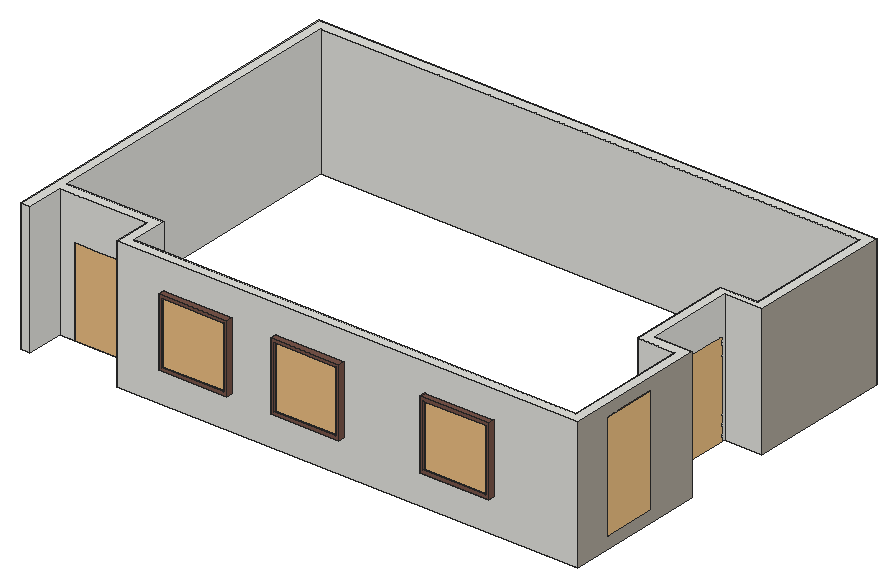
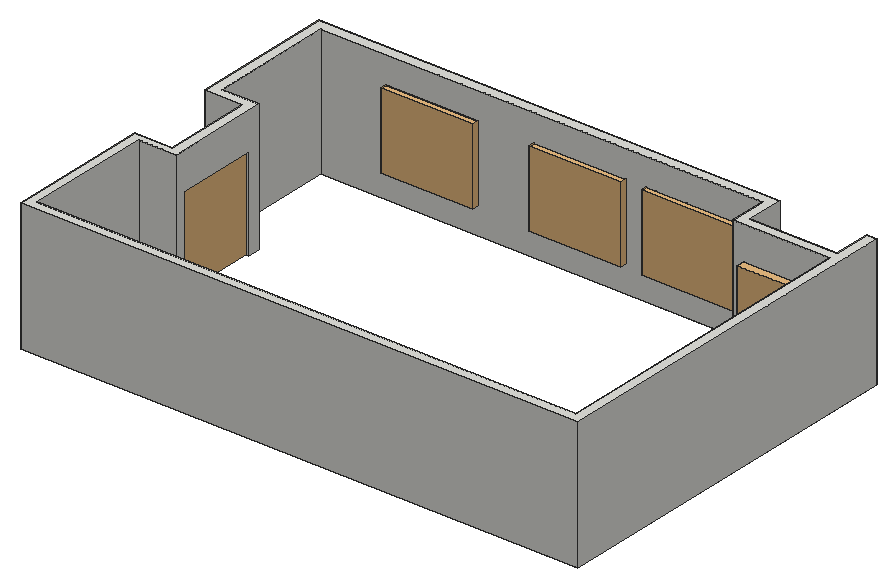
# SketchUp Ruby script. Lengths in inches.
U = 1.inch
M = Sketchup.active_model
def pt(a) = Geom::Point3d.new(a.map { |v| v * U })
def face(e, loops, mat)
  f = e.add_face(loops[0].map { |a| pt(a) })
  loops[1..].each { |l| e.add_face(l.map { |a| pt(a) }).erase! }
  f.material = f.back_material = mat if mat
  f
end
# faces: each face lists its corners as indices into pts; further lists are holes
def faces(e, pts, list, mat = nil) = list.each { |f| face(e, (f[0].is_a?(Array) ? f : [f]).map { |l| l.map { |i| pts[i] } }, mat) }
# xy, xz, yz: faces in a plane at the given z, y or x. An outline is a flat list of corners, or four numbers for a rectangle; further outlines are holes
def ring(l) = l.size == 4 ? [[l[0], l[1]], [l[2], l[1]], [l[2], l[3]], [l[0], l[3]]] : l.each_slice(2).to_a
def flat(e, list, mat, &to3) = list.each { |f| face(e, (f[0].is_a?(Array) ? f : [f]).map { |l| ring(l).map { |u, v| to3.(u, v) } }, mat) }
def xy(e, z, list, mat = nil) = flat(e, list, mat) { |x, y| [x, y, z] }
def xz(e, y, list, mat = nil) = flat(e, list, mat) { |x, z| [x, y, z] }
def yz(e, x, list, mat = nil) = flat(e, list, mat) { |y, z| [x, y, z] }
def lines(e, pts, list) = list.each { |a, b| e.add_line(pt(pts[a]), pt(pts[b])) }
# prism: a flat outline (further loops are holes) pulled along v
def prism(e, loops, v, mat = nil)
  f = face(e, loops, mat); d = Geom::Vector3d.new(v.map { |x| x * U })
  f.pushpull(f.normal.samedirection?(d) ? d.length : -d.length)
end
def box(e, o, s, mat = nil) = prism(e, [[o, [o[0] + s[0], o[1], o[2]], [o[0] + s[0], o[1] + s[1], o[2]], [o[0], o[1] + s[1], o[2]]]], [0, 0, s[2]], mat)
def at(x, y, z, deg = 0) = Geom::Transformation.translation(pt([x, y, z])) * Geom::Transformation.rotation(ORIGIN, Z_AXIS, deg.degrees)
def axes(o, x, y, z) = Geom::Transformation.new([*x, 0, *y, 0, *z, 0, *pt(o).to_a, 1])
def part(name) = M.definitions.add(name)
# library, detail: a bought-in or finely detailed component or shape, given as its bounding box
def library(name, o, s) = part(name).tap { |d| box(d.entities, o, s) }
def detail(e, o, s) = box(e.add_group.entities, o, s)
def put(e, d, t, mat = nil) = e.add_instance(d, t).tap { |i| i.material = mat if mat }
def group(e, t, mat = nil) = e.add_group.tap { |g| g.transformation = t; g.material = mat if mat }.entities
root = M.entities
M.materials.add("1111 AP 9939 Brown seed-N").color = [120, 84, 73]
M.materials.add("Generic").color = [172, 166, 153]
M.materials.add("[Granite Dark Gray]").color = [69, 68, 68]
M.materials.add("[Wood Veneer 01]").color = [120, 70, 37]
c1 = library("Double-hung window 69 in. x 58 in. triple row with mullions",[0,0,-3.59],[62,58,4.59])
c2 = library("Glass Door",[0,0,0],[72,3.54,96])
c3 = library("RIDEAUX \#16",[0,0,0],[103.86,7.74,93.57])
c4 = library("Curtain",[0,0,0],[121.12,7.86,100.24])
c5 = library("SLIDING+GLASS+DOOR",[0,-0.75,0],[72,5.75,80])
c6 = library("Group\#21",[0,0,0],[0.5,51,102])
g1 = group(root,at(36,101.37,167.79))
xy(g1,0,[[0,6,0,366,537,366,537,228,501,228,501,225,492,225,492,234,528,234,528,357,9,357,9,51,24,51,24,42,9,42,9,6],[93,6,93,42,78,42,78,51,102,51,102,15,528,15,528,135,492,135,492,147,501,147,501,144,537,144,537,6]])
xy(g1,33,[[138,0,204,6],[246,0,312,6],[390,0,456,6]],"1111 AP 9939 Brown seed-N")
xy(g1,36,[[141,0,201,15],[249,0,309,15],[393,0,453,15]],"1111 AP 9939 Brown seed-N")
xy(g1,84,[[24,42,78,51]])
xy(g1,90,[[492,147,501,225]])
xy(g1,96,[[141,0,201,15],[249,0,309,15],[393,0,453,15]],"1111 AP 9939 Brown seed-N")
xy(g1,99,[[138,0,204,6],[246,0,312,6],[390,0,456,6]],"1111 AP 9939 Brown seed-N")
xy(g1,126,[[[0,6,9,6,9,42,93,42,93,6,537,6,537,144,501,144,501,228,537,228,537,366,0,366],[102,15,102,51,9,51,9,357,528,357,528,234,492,234,492,135,528,135,528,15]]])
xz(g1,0,[[[138,33,204,99],[141,36,201,96]],[[246,33,312,99],[249,36,309,96]],[[390,33,456,99],[393,36,453,96]]],"1111 AP 9939 Brown seed-N")
xz(g1,6,[[0,0,9,126],[[93,0,537,126],[138,33,204,99],[246,33,312,99],[390,33,456,99]]])
xz(g1,15,[[[102,0,528,126],[141,36,201,96],[249,36,309,96],[393,36,453,96]]])
xz(g1,42,[[9,0,24,0,24,84,78,84,78,0,93,0,93,126,9,126]])
xz(g1,51,[[9,0,9,126,102,126,102,0,78,0,78,84,24,84,24,0]])
xz(g1,135,[[492,0,528,126]])
xz(g1,144,[[501,0,537,126]])
xz(g1,147,[[492,0,501,90]])
xz(g1,225,[[492,0,501,90]])
xz(g1,228,[[501,0,537,126]])
xz(g1,234,[[492,0,528,126]])
xz(g1,357,[[9,0,528,126]])
xz(g1,366,[[0,0,537,126]])
yz(g1,0,[[6,0,366,126]])
yz(g1,9,[[6,0,42,126],[51,0,357,126]])
yz(g1,24,[[42,0,51,84]])
yz(g1,78,[[42,0,51,84]])
yz(g1,93,[[6,0,42,126]])
yz(g1,102,[[15,0,51,126]])
yz(g1,138,[[0,33,6,99]],"[Wood Veneer 01]")
yz(g1,141,[[0,36,15,96]],"1111 AP 9939 Brown seed-N")
yz(g1,201,[[0,36,15,96]],"1111 AP 9939 Brown seed-N")
yz(g1,204,[[0,33,6,99]],"1111 AP 9939 Brown seed-N")
yz(g1,246,[[0,33,6,99]],"1111 AP 9939 Brown seed-N")
yz(g1,249,[[0,36,15,96]],"1111 AP 9939 Brown seed-N")
yz(g1,309,[[0,36,15,96]],"1111 AP 9939 Brown seed-N")
yz(g1,312,[[0,33,6,99]],"1111 AP 9939 Brown seed-N")
yz(g1,390,[[0,33,6,99]],"1111 AP 9939 Brown seed-N")
yz(g1,393,[[0,36,15,96]],"1111 AP 9939 Brown seed-N")
yz(g1,453,[[0,36,15,96]],"1111 AP 9939 Brown seed-N")
yz(g1,456,[[0,33,6,99]],"1111 AP 9939 Brown seed-N")
yz(g1,492,[[135,0,135,126,234,126,234,0,225,0,225,90,147,90,147,0]])
yz(g1,501,[[144,0,147,0,147,90,225,90,225,0,228,0,228,126,144,126]])
yz(g1,528,[[15,0,135,126],[234,0,357,126]])
yz(g1,537,[[[6,0,144,126],[59.76,12,59.53,12.01,59.29,12.01,59.06,12.02,58.82,12.04,58.59,12.06,58.35,12.08,58.12,12.1,57.88,12.125,57.65,12.15,57.42,12.1875,57.18,12.22,56.72,12.3,56.49,12.35,56.26,12.39,56.03,12.44,55.8,12.5,55.57,12.55,55.34,12.61,55.11,12.68,54.89,12.74,54.66,12.81,54.4375,12.88,54.21,12.96,53.99,13.03,53.77,13.11,53.55,13.2,53.33,13.28,52.89,13.46,52.68,13.56,52.46,13.65,52.25,13.75,52.04,13.86,51.83,13.96,51.41,14.18,51.2,14.3,51,14.41,50.6,14.65,50.39,14.78,50.2,14.9,50,15.03,49.8,15.17,49.61,15.3,49.42,15.4375,49.23,15.58,49.04,15.72,48.86,15.86,48.67,16.01,48.49,16.16,48.31,16.3125,48.13,16.47,47.96,16.625,47.78,16.78,47.61,16.94,47.44,17.11,47.27,17.27,47.11,17.44,46.94,17.61,46.78,17.78,46.625,17.96,46.47,18.13,46.3125,18.31,46.16,18.49,46.01,18.67,45.86,18.86,45.72,19.04,45.58,19.23,45.4375,19.42,45.3,19.61,45.17,19.8,45.03,20,44.9,20.2,44.78,20.39,44.65,20.6,44.41,21,44.3,21.2,44.18,21.41,43.96,21.83,43.86,22.04,43.75,22.25,43.65,22.46,43.56,22.68,43.46,22.89,43.28,23.33,43.2,23.55,43.11,23.77,43.03,23.99,42.96,24.21,42.88,24.4375,42.81,24.66,42.74,24.89,42.68,25.11,42.61,25.34,42.55,25.57,42.5,25.8,42.44,26.03,42.39,26.26,42.35,26.49,42.3,26.72,42.22,27.18,42.1875,27.42,42.15,27.65,42.125,27.88,42.1,28.12,42.08,28.35,42.06,28.59,42.04,28.82,42.02,29.06,42.01,29.29,42.01,29.53,42,29.76,42,96.24,42.01,96.47,42.01,96.71,42.02,96.94,42.04,97.18,42.06,97.41,42.08,97.65,42.1,97.88,42.125,98.12,42.15,98.35,42.1875,98.58,42.22,98.82,42.3,99.28,42.35,99.51,42.39,99.74,42.44,99.97,42.5,100.2,42.55,100.43,42.61,100.66,42.68,100.89,42.74,101.11,42.81,101.34,42.88,101.5625,42.96,101.79,43.03,102.01,43.11,102.23,43.2,102.45,43.28,102.67,43.46,103.11,43.56,103.32,43.65,103.54,43.75,103.75,43.86,103.96,43.96,104.17,44.18,104.59,44.3,104.8,44.41,105,44.65,105.4,44.78,105.61,44.9,105.8,45.03,106,45.17,106.2,45.3,106.39,45.4375,106.58,45.58,106.77,45.72,106.96,45.86,107.14,46.01,107.33,46.16,107.51,46.3125,107.69,46.47,107.87,46.625,108.04,46.78,108.22,46.94,108.39,47.11,108.56,47.27,108.73,47.44,108.89,47.61,109.06,47.78,109.22,47.96,109.375,48.13,109.53,48.31,109.6875,48.49,109.84,48.67,109.99,48.86,110.14,49.04,110.28,49.23,110.42,49.42,110.5625,49.61,110.7,49.8,110.83,50,110.97,50.2,111.1,50.39,111.22,50.6,111.35,51,111.59,51.2,111.7,51.41,111.82,51.83,112.04,52.04,112.14,52.25,112.25,52.46,112.35,52.68,112.44,52.89,112.54,53.33,112.72,53.55,112.8,53.77,112.89,53.99,112.97,54.21,113.04,54.4375,113.12,54.66,113.19,54.89,113.26,55.11,113.32,55.34,113.39,55.57,113.45,55.8,113.5,56.03,113.56,56.26,113.61,56.49,113.65,56.72,113.7,57.18,113.78,57.42,113.8125,57.65,113.85,57.88,113.875,58.12,113.9,58.35,113.92,58.59,113.94,58.82,113.96,59.06,113.98,59.29,113.99,59.53,113.99,59.76,114,93,114,93,12]],[228,0,366,126]],"Generic")
yz(g1,537,[[59.76,12,93,12,93,114,59.76,114,59.53,113.99,59.29,113.99,59.06,113.98,58.82,113.96,58.59,113.94,58.35,113.92,58.12,113.9,57.88,113.875,57.65,113.85,57.42,113.8125,57.18,113.78,56.72,113.7,56.49,113.65,56.26,113.61,56.03,113.56,55.8,113.5,55.57,113.45,55.34,113.39,55.11,113.32,54.89,113.26,54.66,113.19,54.4375,113.12,54.21,113.04,53.99,112.97,53.77,112.89,53.55,112.8,53.33,112.72,52.89,112.54,52.68,112.44,52.46,112.35,52.25,112.25,52.04,112.14,51.83,112.04,51.41,111.82,51.2,111.7,51,111.59,50.6,111.35,50.39,111.22,50.2,111.1,50,110.97,49.8,110.83,49.61,110.7,49.42,110.5625,49.23,110.42,49.04,110.28,48.86,110.14,48.67,109.99,48.49,109.84,48.31,109.6875,48.13,109.53,47.96,109.375,47.78,109.22,47.61,109.06,47.44,108.89,47.27,108.73,47.11,108.56,46.94,108.39,46.78,108.22,46.625,108.04,46.47,107.87,46.3125,107.69,46.16,107.51,46.01,107.33,45.86,107.14,45.72,106.96,45.58,106.77,45.4375,106.58,45.3,106.39,45.17,106.2,45.03,106,44.9,105.8,44.78,105.61,44.65,105.4,44.41,105,44.3,104.8,44.18,104.59,43.96,104.17,43.86,103.96,43.75,103.75,43.65,103.54,43.56,103.32,43.46,103.11,43.28,102.67,43.2,102.45,43.11,102.23,43.03,102.01,42.96,101.79,42.88,101.5625,42.81,101.34,42.74,101.11,42.68,100.89,42.61,100.66,42.55,100.43,42.5,100.2,42.44,99.97,42.39,99.74,42.35,99.51,42.3,99.28,42.22,98.82,42.1875,98.58,42.15,98.35,42.125,98.12,42.1,97.88,42.08,97.65,42.06,97.41,42.04,97.18,42.02,96.94,42.01,96.71,42.01,96.47,42,96.24,42,29.76,42.01,29.53,42.01,29.29,42.02,29.06,42.04,28.82,42.06,28.59,42.08,28.35,42.1,28.12,42.125,27.88,42.15,27.65,42.1875,27.42,42.22,27.18,42.3,26.72,42.35,26.49,42.39,26.26,42.44,26.03,42.5,25.8,42.55,25.57,42.61,25.34,42.68,25.11,42.74,24.89,42.81,24.66,42.88,24.4375,42.96,24.21,43.03,23.99,43.11,23.77,43.2,23.55,43.28,23.33,43.46,22.89,43.56,22.68,43.65,22.46,43.75,22.25,43.86,22.04,43.96,21.83,44.18,21.41,44.3,21.2,44.41,21,44.65,20.6,44.78,20.39,44.9,20.2,45.03,20,45.17,19.8,45.3,19.61,45.4375,19.42,45.58,19.23,45.72,19.04,45.86,18.86,46.01,18.67,46.16,18.49,46.3125,18.31,46.47,18.13,46.625,17.96,46.78,17.78,46.94,17.61,47.11,17.44,47.27,17.27,47.44,17.11,47.61,16.94,47.78,16.78,47.96,16.625,48.13,16.47,48.31,16.3125,48.49,16.16,48.67,16.01,48.86,15.86,49.04,15.72,49.23,15.58,49.42,15.4375,49.61,15.3,49.8,15.17,50,15.03,50.2,14.9,50.39,14.78,50.6,14.65,51,14.41,51.2,14.3,51.41,14.18,51.83,13.96,52.04,13.86,52.25,13.75,52.46,13.65,52.68,13.56,52.89,13.46,53.33,13.28,53.55,13.2,53.77,13.11,53.99,13.03,54.21,12.96,54.4375,12.88,54.66,12.81,54.89,12.74,55.11,12.68,55.34,12.61,55.57,12.55,55.8,12.5,56.03,12.44,56.26,12.39,56.49,12.35,56.72,12.3,57.18,12.22,57.42,12.1875,57.65,12.15,57.88,12.125,58.12,12.1,58.35,12.08,58.59,12.06,58.82,12.04,59.06,12.02,59.29,12.01,59.53,12.01]],"[Wood Veneer 01]")
put(g1,c1,axes([201,4.5,36],[-0.96774,0,0],[0,0,1.03448],[0,0.696,0]),"[Granite Dark Gray]")
put(g1,c1,axes([309,4.5,36],[-0.96774,0,0],[0,0,1.03448],[0,0.696,0]),"[Granite Dark Gray]")
put(g1,c1,axes([453,4.5,36],[-0.96774,0,0],[0,0,1.03448],[0,0.696,0]),"[Granite Dark Gray]")
put(g1,c2,axes([24,42,0],[0.75,0,0],[0,0.74,0],[0,0,0.875]))
put(g1,c3,axes([9,51,0],[0.79912,0,0],[0,1,0],[0,0,1]))
put(g1,c4,axes([126.25,15,25.6875],[0.73,0,0],[0,0.73,0],[0,0,0.73]))
put(g1,c4,axes([234.25,15,25.6875],[0.73,0,0],[0,0.73,0],[0,0,0.73]))
put(g1,c4,axes([377,15,25.6875],[0.73,0,0],[0,0.73,0],[0,0,0.73]))
put(g1,c5,axes([496,225,0],[0,-1.08333,0],[1,0,0],[0,0,1.125]))
put(g1,c6,at(537,42,12),"[Wood Veneer 01]")
